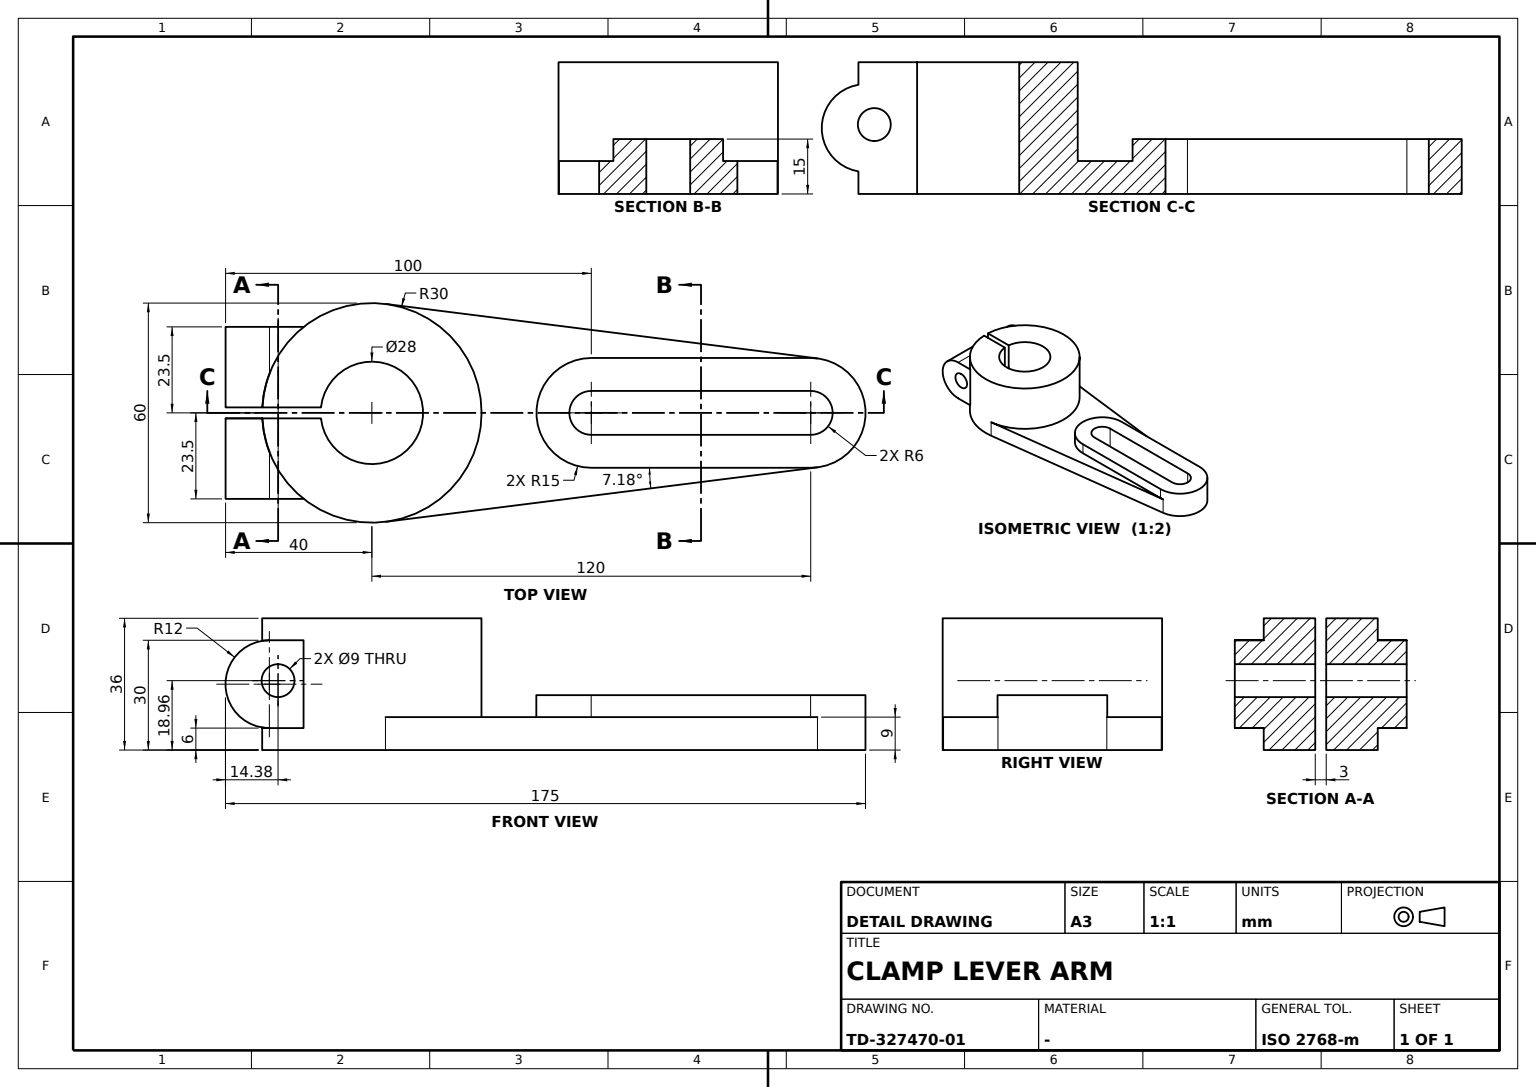
ISO-10303-21;
HEADER;
FILE_DESCRIPTION((''),'2;1');
FILE_NAME('','',(''),(''),'','','');
FILE_SCHEMA(('AUTOMOTIVE_DESIGN'));
ENDSEC;
DATA;
#1=APPLICATION_CONTEXT('');
#2=PRODUCT_CONTEXT('',#1,'mechanical');
#3=PRODUCT('','','',(#2));
#4=PRODUCT_DEFINITION_FORMATION('','',#3);
#5=PRODUCT_DEFINITION_CONTEXT('',#1,'design');
#6=PRODUCT_DEFINITION('','',#4,#5);
#7=PRODUCT_DEFINITION_SHAPE('','',#6);
#8=(LENGTH_UNIT()NAMED_UNIT(*)SI_UNIT(.MILLI.,.METRE.));
#9=(NAMED_UNIT(*)PLANE_ANGLE_UNIT()SI_UNIT($,.RADIAN.));
#10=(NAMED_UNIT(*)SI_UNIT($,.STERADIAN.)SOLID_ANGLE_UNIT());
#11=UNCERTAINTY_MEASURE_WITH_UNIT(LENGTH_MEASURE(0.005),#8,'distance_accuracy_value','');
#12=(GEOMETRIC_REPRESENTATION_CONTEXT(3)GLOBAL_UNCERTAINTY_ASSIGNED_CONTEXT((#11))GLOBAL_UNIT_ASSIGNED_CONTEXT((#8,#9,#10))REPRESENTATION_CONTEXT('',''));
#13=CARTESIAN_POINT('',(-28.,-23.5,30.));
#14=VERTEX_POINT('',#13);
#15=CARTESIAN_POINT('',(-18.648056,-23.5,30.));
#16=VERTEX_POINT('',#15);
#17=CARTESIAN_POINT('',(0.,-23.5,30.));
#18=DIRECTION('',(1.,0.,0.));
#19=VECTOR('',#18,1000.);
#20=LINE('',#17,#19);
#21=EDGE_CURVE('',#14,#16,#20,.T.);
#22=ORIENTED_EDGE('',*,*,#21,.T.);
#23=CARTESIAN_POINT('',(-28.,-10.77033,30.));
#24=VERTEX_POINT('',#23);
#25=CARTESIAN_POINT('',(0.,0.,30.));
#26=DIRECTION('',(0.,0.,1.));
#27=AXIS2_PLACEMENT_3D('',#25,#26,#18);
#28=CIRCLE('',#27,30.);
#29=EDGE_CURVE('',#24,#16,#28,.T.);
#30=ORIENTED_EDGE('',*,*,#29,.F.);
#31=CARTESIAN_POINT('',(-28.,11.75,30.));
#32=DIRECTION('',(0.,1.,0.));
#33=VECTOR('',#32,1000.);
#34=LINE('',#31,#33);
#35=EDGE_CURVE('',#24,#14,#34,.F.);
#36=ORIENTED_EDGE('',*,*,#35,.T.);
#37=EDGE_LOOP('',(#22,#30,#36));
#38=FACE_BOUND('',#37,.T.);
#39=CARTESIAN_POINT('',(-28.,0.,30.));
#40=AXIS2_PLACEMENT_3D('',#39,#26,#18);
#41=PLANE('',#40);
#42=ADVANCED_FACE('',(#38),#41,.T.);
#43=CARTESIAN_POINT('',(3.75,29.764702,9.));
#44=VERTEX_POINT('',#43);
#45=CARTESIAN_POINT('',(3.75,-29.764702,9.));
#46=VERTEX_POINT('',#45);
#47=CARTESIAN_POINT('',(0.,0.,9.));
#48=DIRECTION('',(0.,0.,-1.));
#49=DIRECTION('',(-1.,0.,0.));
#50=AXIS2_PLACEMENT_3D('',#47,#48,#49);
#51=CIRCLE('',#50,30.);
#52=EDGE_CURVE('',#44,#46,#51,.T.);
#53=ORIENTED_EDGE('',*,*,#52,.F.);
#54=CARTESIAN_POINT('',(3.75,29.764702,0.));
#55=VERTEX_POINT('',#54);
#56=CARTESIAN_POINT('',(3.75,29.764702,18.));
#57=VECTOR('',#26,1000.);
#58=LINE('',#56,#57);
#59=EDGE_CURVE('',#55,#44,#58,.T.);
#60=ORIENTED_EDGE('',*,*,#59,.F.);
#61=CARTESIAN_POINT('',(-29.962476,1.5,0.));
#62=VERTEX_POINT('',#61);
#63=CARTESIAN_POINT('',(0.,0.,0.));
#64=AXIS2_PLACEMENT_3D('',#63,#26,#18);
#65=CIRCLE('',#64,30.);
#66=EDGE_CURVE('',#55,#62,#65,.T.);
#67=ORIENTED_EDGE('',*,*,#66,.T.);
#68=CARTESIAN_POINT('',(-29.962476,1.5,6.161559));
#69=VERTEX_POINT('',#68);
#70=CARTESIAN_POINT('',(-29.962476,1.5,6.161558));
#71=LINE('',#70,#57);
#72=EDGE_CURVE('',#69,#62,#71,.F.);
#73=ORIENTED_EDGE('',*,*,#72,.F.);
#74=CARTESIAN_POINT('',(-28.,10.77033,6.));
#75=VERTEX_POINT('',#74);
#76=CARTESIAN_POINT('',(-29.962477,1.5,6.161559));
#77=CARTESIAN_POINT('',(-29.802516,4.695205,6.135042));
#78=CARTESIAN_POINT('',(-29.148715,7.783976,6.));
#79=B_SPLINE_CURVE_WITH_KNOTS('',3,(#76,#77,#78,#74),.UNSPECIFIED.,.F.,.F.,(4,4),(0.,0.009477153),.UNSPECIFIED.);
#80=EDGE_CURVE('',#75,#69,#79,.F.);
#81=ORIENTED_EDGE('',*,*,#80,.F.);
#82=CARTESIAN_POINT('',(-18.648056,23.5,6.));
#83=VERTEX_POINT('',#82);
#84=CARTESIAN_POINT('',(0.,0.,6.));
#85=AXIS2_PLACEMENT_3D('',#84,#26,#18);
#86=CIRCLE('',#85,30.);
#87=EDGE_CURVE('',#83,#75,#86,.T.);
#88=ORIENTED_EDGE('',*,*,#87,.F.);
#89=CARTESIAN_POINT('',(-18.648056,23.5,30.));
#90=VERTEX_POINT('',#89);
#91=LINE('',#82,#57);
#92=EDGE_CURVE('',#83,#90,#91,.T.);
#93=ORIENTED_EDGE('',*,*,#92,.T.);
#94=CARTESIAN_POINT('',(-28.,10.77033,30.));
#95=VERTEX_POINT('',#94);
#96=EDGE_CURVE('',#90,#95,#28,.T.);
#97=ORIENTED_EDGE('',*,*,#96,.T.);
#98=CARTESIAN_POINT('',(-29.962476,1.5,29.838441));
#99=VERTEX_POINT('',#98);
#100=CARTESIAN_POINT('',(-29.962477,1.5,29.838441));
#101=CARTESIAN_POINT('',(-29.802516,4.695205,29.864958));
#102=CARTESIAN_POINT('',(-29.148715,7.783976,30.));
#103=B_SPLINE_CURVE_WITH_KNOTS('',3,(#100,#101,#102,#94),.UNSPECIFIED.,.F.,.F.,(4,4),(0.,0.009477153),.UNSPECIFIED.);
#104=EDGE_CURVE('',#99,#95,#103,.T.);
#105=ORIENTED_EDGE('',*,*,#104,.F.);
#106=CARTESIAN_POINT('',(-29.962477,1.5,36.));
#107=VERTEX_POINT('',#106);
#108=LINE('',#106,#57);
#109=EDGE_CURVE('',#107,#99,#108,.F.);
#110=ORIENTED_EDGE('',*,*,#109,.F.);
#111=CARTESIAN_POINT('',(-29.962477,-1.5,36.));
#112=VERTEX_POINT('',#111);
#113=CARTESIAN_POINT('',(0.,0.,36.));
#114=AXIS2_PLACEMENT_3D('',#113,#26,#18);
#115=CIRCLE('',#114,30.);
#116=EDGE_CURVE('',#112,#107,#115,.T.);
#117=ORIENTED_EDGE('',*,*,#116,.F.);
#118=CARTESIAN_POINT('',(-29.962477,-1.5,29.838441));
#119=VERTEX_POINT('',#118);
#120=LINE('',#111,#57);
#121=EDGE_CURVE('',#112,#119,#120,.F.);
#122=ORIENTED_EDGE('',*,*,#121,.T.);
#123=CARTESIAN_POINT('',(-29.802516,-4.695205,29.864958));
#124=CARTESIAN_POINT('',(-29.148715,-7.783976,30.));
#125=B_SPLINE_CURVE_WITH_KNOTS('',3,(#118,#123,#124,#23),.UNSPECIFIED.,.F.,.F.,(4,4),(0.,0.009477153),.UNSPECIFIED.);
#126=EDGE_CURVE('',#24,#119,#125,.F.);
#127=ORIENTED_EDGE('',*,*,#126,.F.);
#128=ORIENTED_EDGE('',*,*,#29,.T.);
#129=CARTESIAN_POINT('',(-18.648056,-23.5,6.));
#130=VERTEX_POINT('',#129);
#131=LINE('',#129,#57);
#132=EDGE_CURVE('',#130,#16,#131,.T.);
#133=ORIENTED_EDGE('',*,*,#132,.F.);
#134=CARTESIAN_POINT('',(-28.,-10.77033,6.));
#135=VERTEX_POINT('',#134);
#136=EDGE_CURVE('',#135,#130,#86,.T.);
#137=ORIENTED_EDGE('',*,*,#136,.F.);
#138=CARTESIAN_POINT('',(-29.962476,-1.5,6.161559));
#139=VERTEX_POINT('',#138);
#140=CARTESIAN_POINT('',(-29.962477,-1.5,6.161559));
#141=CARTESIAN_POINT('',(-29.802516,-4.695205,6.135042));
#142=CARTESIAN_POINT('',(-29.148715,-7.783976,6.));
#143=B_SPLINE_CURVE_WITH_KNOTS('',3,(#140,#141,#142,#134),.UNSPECIFIED.,.F.,.F.,(4,4),(0.,0.009477153),.UNSPECIFIED.);
#144=EDGE_CURVE('',#139,#135,#143,.T.);
#145=ORIENTED_EDGE('',*,*,#144,.F.);
#146=CARTESIAN_POINT('',(-29.962476,-1.5,0.));
#147=VERTEX_POINT('',#146);
#148=CARTESIAN_POINT('',(-29.962476,-1.5,6.161558));
#149=LINE('',#148,#57);
#150=EDGE_CURVE('',#139,#147,#149,.F.);
#151=ORIENTED_EDGE('',*,*,#150,.T.);
#152=CARTESIAN_POINT('',(3.75,-29.764702,0.));
#153=VERTEX_POINT('',#152);
#154=EDGE_CURVE('',#147,#153,#65,.T.);
#155=ORIENTED_EDGE('',*,*,#154,.T.);
#156=CARTESIAN_POINT('',(3.75,-29.764702,18.));
#157=LINE('',#156,#57);
#158=EDGE_CURVE('',#153,#46,#157,.T.);
#159=ORIENTED_EDGE('',*,*,#158,.T.);
#160=EDGE_LOOP('',(#53,#60,#67,#73,#81,#88,#93,#97,#105,#110,#117,#122,#127,#128,#133,#137,#145,#151,#155,#159));
#161=FACE_BOUND('',#160,.T.);
#162=CARTESIAN_POINT('',(0.,0.,18.));
#163=AXIS2_PLACEMENT_3D('',#162,#26,#18);
#164=CYLINDRICAL_SURFACE('',#163,30.);
#165=ADVANCED_FACE('',(#161),#164,.T.);
#166=CARTESIAN_POINT('',(-28.,-23.5,6.));
#167=VERTEX_POINT('',#166);
#168=CARTESIAN_POINT('',(-28.,-23.5,18.));
#169=AXIS2_PLACEMENT_3D('',#168,#32,#26);
#170=CIRCLE('',#169,12.);
#171=EDGE_CURVE('',#167,#14,#170,.T.);
#172=ORIENTED_EDGE('',*,*,#171,.T.);
#173=ORIENTED_EDGE('',*,*,#35,.F.);
#174=ORIENTED_EDGE('',*,*,#126,.T.);
#175=CARTESIAN_POINT('',(-28.,-1.5,18.));
#176=AXIS2_PLACEMENT_3D('',#175,#32,#26);
#177=CIRCLE('',#176,12.);
#178=EDGE_CURVE('',#139,#119,#177,.T.);
#179=ORIENTED_EDGE('',*,*,#178,.F.);
#180=ORIENTED_EDGE('',*,*,#144,.T.);
#181=CARTESIAN_POINT('',(-28.,11.75,6.));
#182=LINE('',#181,#33);
#183=EDGE_CURVE('',#135,#167,#182,.F.);
#184=ORIENTED_EDGE('',*,*,#183,.T.);
#185=EDGE_LOOP('',(#172,#173,#174,#179,#180,#184));
#186=FACE_BOUND('',#185,.T.);
#187=CARTESIAN_POINT('',(-28.,11.75,18.));
#188=AXIS2_PLACEMENT_3D('',#187,#32,#49);
#189=CYLINDRICAL_SURFACE('',#188,12.);
#190=ADVANCED_FACE('',(#186),#189,.T.);
#191=CARTESIAN_POINT('',(120.,-15.,9.));
#192=VERTEX_POINT('',#191);
#193=CARTESIAN_POINT('',(120.,-15.,15.));
#194=VERTEX_POINT('',#193);
#195=CARTESIAN_POINT('',(120.,-15.,7.5));
#196=LINE('',#195,#57);
#197=EDGE_CURVE('',#192,#194,#196,.T.);
#198=ORIENTED_EDGE('',*,*,#197,.F.);
#199=CARTESIAN_POINT('',(121.875,-14.882351,9.));
#200=VERTEX_POINT('',#199);
#201=CARTESIAN_POINT('',(120.,0.,9.));
#202=AXIS2_PLACEMENT_3D('',#201,#48,#49);
#203=CIRCLE('',#202,15.);
#204=EDGE_CURVE('',#200,#192,#203,.T.);
#205=ORIENTED_EDGE('',*,*,#204,.F.);
#206=CARTESIAN_POINT('',(121.875,-14.882351,0.));
#207=VERTEX_POINT('',#206);
#208=CARTESIAN_POINT('',(121.875,-14.882351,7.5));
#209=LINE('',#208,#57);
#210=EDGE_CURVE('',#207,#200,#209,.T.);
#211=ORIENTED_EDGE('',*,*,#210,.F.);
#212=CARTESIAN_POINT('',(121.875,14.882351,0.));
#213=VERTEX_POINT('',#212);
#214=CARTESIAN_POINT('',(120.,0.,0.));
#215=AXIS2_PLACEMENT_3D('',#214,#26,#18);
#216=CIRCLE('',#215,15.);
#217=EDGE_CURVE('',#207,#213,#216,.T.);
#218=ORIENTED_EDGE('',*,*,#217,.T.);
#219=CARTESIAN_POINT('',(121.875,14.882351,9.));
#220=VERTEX_POINT('',#219);
#221=CARTESIAN_POINT('',(121.875,14.882351,7.5));
#222=LINE('',#221,#57);
#223=EDGE_CURVE('',#213,#220,#222,.T.);
#224=ORIENTED_EDGE('',*,*,#223,.T.);
#225=CARTESIAN_POINT('',(120.,15.,9.));
#226=VERTEX_POINT('',#225);
#227=EDGE_CURVE('',#226,#220,#203,.T.);
#228=ORIENTED_EDGE('',*,*,#227,.F.);
#229=CARTESIAN_POINT('',(120.,15.,15.));
#230=VERTEX_POINT('',#229);
#231=CARTESIAN_POINT('',(120.,15.,7.5));
#232=LINE('',#231,#57);
#233=EDGE_CURVE('',#226,#230,#232,.T.);
#234=ORIENTED_EDGE('',*,*,#233,.T.);
#235=CARTESIAN_POINT('',(120.,0.,15.));
#236=AXIS2_PLACEMENT_3D('',#235,#26,#18);
#237=CIRCLE('',#236,15.);
#238=EDGE_CURVE('',#194,#230,#237,.T.);
#239=ORIENTED_EDGE('',*,*,#238,.F.);
#240=EDGE_LOOP('',(#198,#205,#211,#218,#224,#228,#234,#239));
#241=FACE_BOUND('',#240,.T.);
#242=CARTESIAN_POINT('',(120.,0.,7.5));
#243=AXIS2_PLACEMENT_3D('',#242,#26,#18);
#244=CYLINDRICAL_SURFACE('',#243,15.);
#245=ADVANCED_FACE('',(#241),#244,.T.);
#246=ORIENTED_EDGE('',*,*,#227,.T.);
#247=DIRECTION('',(0.992156742,-0.125,0.));
#248=VECTOR('',#247,1000.);
#249=LINE('',#43,#248);
#250=EDGE_CURVE('',#44,#220,#249,.T.);
#251=ORIENTED_EDGE('',*,*,#250,.F.);
#252=ORIENTED_EDGE('',*,*,#52,.T.);
#253=DIRECTION('',(0.992156742,0.125,0.));
#254=VECTOR('',#253,1000.);
#255=LINE('',#45,#254);
#256=EDGE_CURVE('',#46,#200,#255,.T.);
#257=ORIENTED_EDGE('',*,*,#256,.T.);
#258=ORIENTED_EDGE('',*,*,#204,.T.);
#259=CARTESIAN_POINT('',(60.,-15.,9.));
#260=VERTEX_POINT('',#259);
#261=CARTESIAN_POINT('',(0.,-15.,9.));
#262=LINE('',#261,#19);
#263=EDGE_CURVE('',#260,#192,#262,.T.);
#264=ORIENTED_EDGE('',*,*,#263,.F.);
#265=CARTESIAN_POINT('',(60.,15.,9.));
#266=VERTEX_POINT('',#265);
#267=CARTESIAN_POINT('',(60.,0.,9.));
#268=AXIS2_PLACEMENT_3D('',#267,#48,#49);
#269=CIRCLE('',#268,15.);
#270=EDGE_CURVE('',#260,#266,#269,.T.);
#271=ORIENTED_EDGE('',*,*,#270,.T.);
#272=CARTESIAN_POINT('',(0.,15.,9.));
#273=VECTOR('',#49,1000.);
#274=LINE('',#272,#273);
#275=EDGE_CURVE('',#226,#266,#274,.T.);
#276=ORIENTED_EDGE('',*,*,#275,.F.);
#277=EDGE_LOOP('',(#246,#251,#252,#257,#258,#264,#271,#276));
#278=FACE_BOUND('',#277,.T.);
#279=AXIS2_PLACEMENT_3D('',#47,#48,#18);
#280=PLANE('',#279);
#281=ADVANCED_FACE('',(#278),#280,.F.);
#282=CARTESIAN_POINT('',(-13.919411,1.5,36.));
#283=VERTEX_POINT('',#282);
#284=CARTESIAN_POINT('',(-13.919411,1.5,0.));
#285=VERTEX_POINT('',#284);
#286=CARTESIAN_POINT('',(-13.919411,1.5,30.));
#287=LINE('',#286,#57);
#288=EDGE_CURVE('',#283,#285,#287,.F.);
#289=ORIENTED_EDGE('',*,*,#288,.T.);
#290=CARTESIAN_POINT('',(-13.919411,-1.5,0.));
#291=VERTEX_POINT('',#290);
#292=CIRCLE('',#64,14.);
#293=EDGE_CURVE('',#291,#285,#292,.T.);
#294=ORIENTED_EDGE('',*,*,#293,.F.);
#295=CARTESIAN_POINT('',(-13.919411,-1.5,36.));
#296=VERTEX_POINT('',#295);
#297=CARTESIAN_POINT('',(-13.919411,-1.5,30.));
#298=LINE('',#297,#57);
#299=EDGE_CURVE('',#291,#296,#298,.T.);
#300=ORIENTED_EDGE('',*,*,#299,.T.);
#301=CIRCLE('',#114,14.);
#302=EDGE_CURVE('',#296,#283,#301,.T.);
#303=ORIENTED_EDGE('',*,*,#302,.T.);
#304=EDGE_LOOP('',(#289,#294,#300,#303));
#305=FACE_BOUND('',#304,.T.);
#306=CARTESIAN_POINT('',(0.,0.,17.34));
#307=AXIS2_PLACEMENT_3D('',#306,#26,#18);
#308=CYLINDRICAL_SURFACE('',#307,14.);
#309=ADVANCED_FACE('',(#305),#308,.F.);
#310=CARTESIAN_POINT('',(120.,-6.,0.));
#311=VERTEX_POINT('',#310);
#312=CARTESIAN_POINT('',(120.,6.,0.));
#313=VERTEX_POINT('',#312);
#314=CIRCLE('',#215,6.);
#315=EDGE_CURVE('',#311,#313,#314,.T.);
#316=ORIENTED_EDGE('',*,*,#315,.T.);
#317=CARTESIAN_POINT('',(60.,6.,0.));
#318=VERTEX_POINT('',#317);
#319=CARTESIAN_POINT('',(0.,6.,0.));
#320=LINE('',#319,#19);
#321=EDGE_CURVE('',#318,#313,#320,.T.);
#322=ORIENTED_EDGE('',*,*,#321,.F.);
#323=CARTESIAN_POINT('',(60.,-6.,0.));
#324=VERTEX_POINT('',#323);
#325=CARTESIAN_POINT('',(60.,0.,0.));
#326=AXIS2_PLACEMENT_3D('',#325,#26,#18);
#327=CIRCLE('',#326,6.);
#328=EDGE_CURVE('',#318,#324,#327,.T.);
#329=ORIENTED_EDGE('',*,*,#328,.T.);
#330=CARTESIAN_POINT('',(0.,-6.,0.));
#331=LINE('',#330,#273);
#332=EDGE_CURVE('',#311,#324,#331,.T.);
#333=ORIENTED_EDGE('',*,*,#332,.F.);
#334=EDGE_LOOP('',(#316,#322,#329,#333));
#335=FACE_BOUND('',#334,.T.);
#336=LINE('',#152,#254);
#337=EDGE_CURVE('',#153,#207,#336,.T.);
#338=ORIENTED_EDGE('',*,*,#337,.F.);
#339=ORIENTED_EDGE('',*,*,#154,.F.);
#340=CARTESIAN_POINT('',(0.,-1.5,0.));
#341=LINE('',#340,#273);
#342=EDGE_CURVE('',#291,#147,#341,.T.);
#343=ORIENTED_EDGE('',*,*,#342,.F.);
#344=ORIENTED_EDGE('',*,*,#293,.T.);
#345=LINE('',#284,#273);
#346=EDGE_CURVE('',#285,#62,#345,.T.);
#347=ORIENTED_EDGE('',*,*,#346,.T.);
#348=ORIENTED_EDGE('',*,*,#66,.F.);
#349=LINE('',#54,#248);
#350=EDGE_CURVE('',#55,#213,#349,.T.);
#351=ORIENTED_EDGE('',*,*,#350,.T.);
#352=ORIENTED_EDGE('',*,*,#217,.F.);
#353=EDGE_LOOP('',(#338,#339,#343,#344,#347,#348,#351,#352));
#354=FACE_BOUND('',#353,.T.);
#355=PLANE('',#64);
#356=ADVANCED_FACE('',(#335,#354),#355,.F.);
#357=CARTESIAN_POINT('',(-25.620803,23.5,23.464319));
#358=VERTEX_POINT('',#357);
#359=CARTESIAN_POINT('',(-25.620803,23.5,18.964319));
#360=AXIS2_PLACEMENT_3D('',#359,#32,#26);
#361=CIRCLE('',#360,4.5);
#362=EDGE_CURVE('',#358,#358,#361,.T.);
#363=ORIENTED_EDGE('',*,*,#362,.T.);
#364=EDGE_LOOP('',(#363));
#365=FACE_BOUND('',#364,.T.);
#366=CARTESIAN_POINT('',(-25.620803,1.5,14.464319));
#367=VERTEX_POINT('',#366);
#368=CARTESIAN_POINT('',(-25.620803,1.5,18.964319));
#369=DIRECTION('',(0.,-1.,0.));
#370=AXIS2_PLACEMENT_3D('',#368,#369,#48);
#371=CIRCLE('',#370,4.5);
#372=EDGE_CURVE('',#367,#367,#371,.T.);
#373=ORIENTED_EDGE('',*,*,#372,.T.);
#374=EDGE_LOOP('',(#373));
#375=FACE_BOUND('',#374,.T.);
#376=CARTESIAN_POINT('',(-25.620803,3.91,18.964319));
#377=AXIS2_PLACEMENT_3D('',#376,#369,#18);
#378=CYLINDRICAL_SURFACE('',#377,4.5);
#379=ADVANCED_FACE('',(#365,#375),#378,.F.);
#380=CARTESIAN_POINT('',(60.,15.,15.));
#381=VERTEX_POINT('',#380);
#382=CARTESIAN_POINT('',(60.,-15.,15.));
#383=VERTEX_POINT('',#382);
#384=CARTESIAN_POINT('',(60.,0.,15.));
#385=AXIS2_PLACEMENT_3D('',#384,#26,#18);
#386=CIRCLE('',#385,15.);
#387=EDGE_CURVE('',#381,#383,#386,.T.);
#388=ORIENTED_EDGE('',*,*,#387,.F.);
#389=CARTESIAN_POINT('',(60.,15.,7.5));
#390=LINE('',#389,#57);
#391=EDGE_CURVE('',#266,#381,#390,.T.);
#392=ORIENTED_EDGE('',*,*,#391,.F.);
#393=ORIENTED_EDGE('',*,*,#270,.F.);
#394=CARTESIAN_POINT('',(60.,-15.,7.5));
#395=LINE('',#394,#57);
#396=EDGE_CURVE('',#260,#383,#395,.T.);
#397=ORIENTED_EDGE('',*,*,#396,.T.);
#398=EDGE_LOOP('',(#388,#392,#393,#397));
#399=FACE_BOUND('',#398,.T.);
#400=CARTESIAN_POINT('',(60.,0.,7.5));
#401=AXIS2_PLACEMENT_3D('',#400,#26,#18);
#402=CYLINDRICAL_SURFACE('',#401,15.);
#403=ADVANCED_FACE('',(#399),#402,.T.);
#404=CARTESIAN_POINT('',(60.,6.,15.));
#405=VERTEX_POINT('',#404);
#406=CARTESIAN_POINT('',(60.,6.,7.5));
#407=LINE('',#406,#57);
#408=EDGE_CURVE('',#318,#405,#407,.T.);
#409=ORIENTED_EDGE('',*,*,#408,.T.);
#410=CARTESIAN_POINT('',(60.,-6.,15.));
#411=VERTEX_POINT('',#410);
#412=CIRCLE('',#385,6.);
#413=EDGE_CURVE('',#405,#411,#412,.T.);
#414=ORIENTED_EDGE('',*,*,#413,.T.);
#415=CARTESIAN_POINT('',(60.,-6.,7.5));
#416=LINE('',#415,#57);
#417=EDGE_CURVE('',#324,#411,#416,.T.);
#418=ORIENTED_EDGE('',*,*,#417,.F.);
#419=ORIENTED_EDGE('',*,*,#328,.F.);
#420=EDGE_LOOP('',(#409,#414,#418,#419));
#421=FACE_BOUND('',#420,.T.);
#422=CYLINDRICAL_SURFACE('',#401,6.);
#423=ADVANCED_FACE('',(#421),#422,.F.);
#424=CARTESIAN_POINT('',(120.,-6.,15.));
#425=VERTEX_POINT('',#424);
#426=CARTESIAN_POINT('',(0.,-6.,15.));
#427=LINE('',#426,#273);
#428=EDGE_CURVE('',#425,#411,#427,.T.);
#429=ORIENTED_EDGE('',*,*,#428,.F.);
#430=CARTESIAN_POINT('',(120.,-6.,7.5));
#431=LINE('',#430,#57);
#432=EDGE_CURVE('',#311,#425,#431,.T.);
#433=ORIENTED_EDGE('',*,*,#432,.F.);
#434=ORIENTED_EDGE('',*,*,#332,.T.);
#435=ORIENTED_EDGE('',*,*,#417,.T.);
#436=EDGE_LOOP('',(#429,#433,#434,#435));
#437=FACE_BOUND('',#436,.T.);
#438=AXIS2_PLACEMENT_3D('',#310,#32,#49);
#439=PLANE('',#438);
#440=ADVANCED_FACE('',(#437),#439,.T.);
#441=ORIENTED_EDGE('',*,*,#362,.F.);
#442=EDGE_LOOP('',(#441));
#443=FACE_BOUND('',#442,.T.);
#444=ORIENTED_EDGE('',*,*,#92,.F.);
#445=CARTESIAN_POINT('',(-28.,23.5,6.));
#446=VERTEX_POINT('',#445);
#447=CARTESIAN_POINT('',(0.,23.5,6.));
#448=LINE('',#447,#19);
#449=EDGE_CURVE('',#446,#83,#448,.T.);
#450=ORIENTED_EDGE('',*,*,#449,.F.);
#451=CARTESIAN_POINT('',(-28.,23.5,30.));
#452=VERTEX_POINT('',#451);
#453=CARTESIAN_POINT('',(-28.,23.5,18.));
#454=AXIS2_PLACEMENT_3D('',#453,#32,#26);
#455=CIRCLE('',#454,12.);
#456=EDGE_CURVE('',#446,#452,#455,.T.);
#457=ORIENTED_EDGE('',*,*,#456,.T.);
#458=CARTESIAN_POINT('',(0.,23.5,30.));
#459=LINE('',#458,#19);
#460=EDGE_CURVE('',#452,#90,#459,.T.);
#461=ORIENTED_EDGE('',*,*,#460,.T.);
#462=EDGE_LOOP('',(#444,#450,#457,#461));
#463=FACE_BOUND('',#462,.T.);
#464=CARTESIAN_POINT('',(0.,23.5,0.));
#465=AXIS2_PLACEMENT_3D('',#464,#32,#49);
#466=PLANE('',#465);
#467=ADVANCED_FACE('',(#443,#463),#466,.T.);
#468=ORIENTED_EDGE('',*,*,#396,.F.);
#469=ORIENTED_EDGE('',*,*,#263,.T.);
#470=ORIENTED_EDGE('',*,*,#197,.T.);
#471=CARTESIAN_POINT('',(0.,-15.,15.));
#472=LINE('',#471,#273);
#473=EDGE_CURVE('',#194,#383,#472,.T.);
#474=ORIENTED_EDGE('',*,*,#473,.T.);
#475=EDGE_LOOP('',(#468,#469,#470,#474));
#476=FACE_BOUND('',#475,.T.);
#477=CARTESIAN_POINT('',(120.,-15.,0.));
#478=AXIS2_PLACEMENT_3D('',#477,#32,#49);
#479=PLANE('',#478);
#480=ADVANCED_FACE('',(#476),#479,.F.);
#481=CARTESIAN_POINT('',(0.,-23.5,6.));
#482=LINE('',#481,#19);
#483=EDGE_CURVE('',#167,#130,#482,.T.);
#484=ORIENTED_EDGE('',*,*,#483,.F.);
#485=ORIENTED_EDGE('',*,*,#183,.F.);
#486=ORIENTED_EDGE('',*,*,#136,.T.);
#487=EDGE_LOOP('',(#484,#485,#486));
#488=FACE_BOUND('',#487,.T.);
#489=CARTESIAN_POINT('',(-28.,0.,6.));
#490=AXIS2_PLACEMENT_3D('',#489,#26,#18);
#491=PLANE('',#490);
#492=ADVANCED_FACE('',(#488),#491,.F.);
#493=ORIENTED_EDGE('',*,*,#408,.F.);
#494=ORIENTED_EDGE('',*,*,#321,.T.);
#495=CARTESIAN_POINT('',(120.,6.,15.));
#496=VERTEX_POINT('',#495);
#497=CARTESIAN_POINT('',(120.,6.,7.5));
#498=LINE('',#497,#57);
#499=EDGE_CURVE('',#313,#496,#498,.T.);
#500=ORIENTED_EDGE('',*,*,#499,.T.);
#501=CARTESIAN_POINT('',(0.,6.,15.));
#502=LINE('',#501,#19);
#503=EDGE_CURVE('',#405,#496,#502,.T.);
#504=ORIENTED_EDGE('',*,*,#503,.F.);
#505=EDGE_LOOP('',(#493,#494,#500,#504));
#506=FACE_BOUND('',#505,.T.);
#507=AXIS2_PLACEMENT_3D('',#317,#369,#18);
#508=PLANE('',#507);
#509=ADVANCED_FACE('',(#506),#508,.T.);
#510=CARTESIAN_POINT('',(-25.620803,-1.5,23.464319));
#511=VERTEX_POINT('',#510);
#512=CARTESIAN_POINT('',(-25.620803,-1.5,18.964319));
#513=AXIS2_PLACEMENT_3D('',#512,#32,#26);
#514=CIRCLE('',#513,4.5);
#515=EDGE_CURVE('',#511,#511,#514,.T.);
#516=ORIENTED_EDGE('',*,*,#515,.T.);
#517=EDGE_LOOP('',(#516));
#518=FACE_BOUND('',#517,.T.);
#519=CARTESIAN_POINT('',(-25.620803,-23.5,23.464319));
#520=VERTEX_POINT('',#519);
#521=CARTESIAN_POINT('',(-25.620803,-23.5,18.964319));
#522=AXIS2_PLACEMENT_3D('',#521,#32,#26);
#523=CIRCLE('',#522,4.5);
#524=EDGE_CURVE('',#520,#520,#523,.F.);
#525=ORIENTED_EDGE('',*,*,#524,.T.);
#526=EDGE_LOOP('',(#525));
#527=FACE_BOUND('',#526,.T.);
#528=ADVANCED_FACE('',(#518,#527),#378,.F.);
#529=ORIENTED_EDGE('',*,*,#233,.F.);
#530=ORIENTED_EDGE('',*,*,#275,.T.);
#531=ORIENTED_EDGE('',*,*,#391,.T.);
#532=CARTESIAN_POINT('',(0.,15.,15.));
#533=LINE('',#532,#19);
#534=EDGE_CURVE('',#381,#230,#533,.T.);
#535=ORIENTED_EDGE('',*,*,#534,.T.);
#536=EDGE_LOOP('',(#529,#530,#531,#535));
#537=FACE_BOUND('',#536,.T.);
#538=CARTESIAN_POINT('',(60.,15.,0.));
#539=AXIS2_PLACEMENT_3D('',#538,#369,#18);
#540=PLANE('',#539);
#541=ADVANCED_FACE('',(#537),#540,.F.);
#542=ORIENTED_EDGE('',*,*,#515,.F.);
#543=EDGE_LOOP('',(#542));
#544=FACE_BOUND('',#543,.T.);
#545=ORIENTED_EDGE('',*,*,#299,.F.);
#546=ORIENTED_EDGE('',*,*,#342,.T.);
#547=ORIENTED_EDGE('',*,*,#150,.F.);
#548=ORIENTED_EDGE('',*,*,#178,.T.);
#549=ORIENTED_EDGE('',*,*,#121,.F.);
#550=CARTESIAN_POINT('',(-50.,-1.5,36.));
#551=LINE('',#550,#19);
#552=EDGE_CURVE('',#112,#296,#551,.T.);
#553=ORIENTED_EDGE('',*,*,#552,.T.);
#554=EDGE_LOOP('',(#545,#546,#547,#548,#549,#553));
#555=FACE_BOUND('',#554,.T.);
#556=AXIS2_PLACEMENT_3D('',#550,#32,#18);
#557=PLANE('',#556);
#558=ADVANCED_FACE('',(#544,#555),#557,.T.);
#559=ORIENTED_EDGE('',*,*,#483,.T.);
#560=ORIENTED_EDGE('',*,*,#132,.T.);
#561=ORIENTED_EDGE('',*,*,#21,.F.);
#562=ORIENTED_EDGE('',*,*,#171,.F.);
#563=EDGE_LOOP('',(#559,#560,#561,#562));
#564=FACE_BOUND('',#563,.T.);
#565=ORIENTED_EDGE('',*,*,#524,.F.);
#566=EDGE_LOOP('',(#565));
#567=FACE_BOUND('',#566,.T.);
#568=CARTESIAN_POINT('',(0.,-23.5,0.));
#569=AXIS2_PLACEMENT_3D('',#568,#32,#49);
#570=PLANE('',#569);
#571=ADVANCED_FACE('',(#564,#567),#570,.F.);
#572=ORIENTED_EDGE('',*,*,#96,.F.);
#573=ORIENTED_EDGE('',*,*,#460,.F.);
#574=EDGE_CURVE('',#95,#452,#34,.T.);
#575=ORIENTED_EDGE('',*,*,#574,.F.);
#576=EDGE_LOOP('',(#572,#573,#575));
#577=FACE_BOUND('',#576,.T.);
#578=ADVANCED_FACE('',(#577),#41,.T.);
#579=ORIENTED_EDGE('',*,*,#387,.T.);
#580=ORIENTED_EDGE('',*,*,#473,.F.);
#581=ORIENTED_EDGE('',*,*,#238,.T.);
#582=ORIENTED_EDGE('',*,*,#534,.F.);
#583=EDGE_LOOP('',(#579,#580,#581,#582));
#584=FACE_BOUND('',#583,.T.);
#585=CIRCLE('',#236,6.);
#586=EDGE_CURVE('',#425,#496,#585,.T.);
#587=ORIENTED_EDGE('',*,*,#586,.F.);
#588=ORIENTED_EDGE('',*,*,#428,.T.);
#589=ORIENTED_EDGE('',*,*,#413,.F.);
#590=ORIENTED_EDGE('',*,*,#503,.T.);
#591=EDGE_LOOP('',(#587,#588,#589,#590));
#592=FACE_BOUND('',#591,.T.);
#593=CARTESIAN_POINT('',(0.,0.,15.));
#594=AXIS2_PLACEMENT_3D('',#593,#26,#18);
#595=PLANE('',#594);
#596=ADVANCED_FACE('',(#584,#592),#595,.T.);
#597=ORIENTED_EDGE('',*,*,#586,.T.);
#598=ORIENTED_EDGE('',*,*,#499,.F.);
#599=ORIENTED_EDGE('',*,*,#315,.F.);
#600=ORIENTED_EDGE('',*,*,#432,.T.);
#601=EDGE_LOOP('',(#597,#598,#599,#600));
#602=FACE_BOUND('',#601,.T.);
#603=CYLINDRICAL_SURFACE('',#243,6.);
#604=ADVANCED_FACE('',(#602),#603,.F.);
#605=ORIENTED_EDGE('',*,*,#210,.T.);
#606=ORIENTED_EDGE('',*,*,#256,.F.);
#607=ORIENTED_EDGE('',*,*,#158,.F.);
#608=ORIENTED_EDGE('',*,*,#337,.T.);
#609=EDGE_LOOP('',(#605,#606,#607,#608));
#610=FACE_BOUND('',#609,.T.);
#611=DIRECTION('',(0.125,-0.992156742,0.));
#612=AXIS2_PLACEMENT_3D('',#152,#611,#253);
#613=PLANE('',#612);
#614=ADVANCED_FACE('',(#610),#613,.T.);
#615=ORIENTED_EDGE('',*,*,#302,.F.);
#616=ORIENTED_EDGE('',*,*,#552,.F.);
#617=ORIENTED_EDGE('',*,*,#116,.T.);
#618=LINE('',#282,#273);
#619=EDGE_CURVE('',#283,#107,#618,.T.);
#620=ORIENTED_EDGE('',*,*,#619,.F.);
#621=EDGE_LOOP('',(#615,#616,#617,#620));
#622=FACE_BOUND('',#621,.T.);
#623=PLANE('',#114);
#624=ADVANCED_FACE('',(#622),#623,.T.);
#625=CARTESIAN_POINT('',(-28.,1.5,18.));
#626=AXIS2_PLACEMENT_3D('',#625,#369,#48);
#627=CIRCLE('',#626,12.);
#628=EDGE_CURVE('',#99,#69,#627,.T.);
#629=ORIENTED_EDGE('',*,*,#628,.F.);
#630=ORIENTED_EDGE('',*,*,#104,.T.);
#631=ORIENTED_EDGE('',*,*,#574,.T.);
#632=ORIENTED_EDGE('',*,*,#456,.F.);
#633=EDGE_CURVE('',#75,#446,#182,.T.);
#634=ORIENTED_EDGE('',*,*,#633,.F.);
#635=ORIENTED_EDGE('',*,*,#80,.T.);
#636=EDGE_LOOP('',(#629,#630,#631,#632,#634,#635));
#637=FACE_BOUND('',#636,.T.);
#638=ADVANCED_FACE('',(#637),#189,.T.);
#639=ORIENTED_EDGE('',*,*,#449,.T.);
#640=ORIENTED_EDGE('',*,*,#87,.T.);
#641=ORIENTED_EDGE('',*,*,#633,.T.);
#642=EDGE_LOOP('',(#639,#640,#641));
#643=FACE_BOUND('',#642,.T.);
#644=ADVANCED_FACE('',(#643),#491,.F.);
#645=ORIENTED_EDGE('',*,*,#59,.T.);
#646=ORIENTED_EDGE('',*,*,#250,.T.);
#647=ORIENTED_EDGE('',*,*,#223,.F.);
#648=ORIENTED_EDGE('',*,*,#350,.F.);
#649=EDGE_LOOP('',(#645,#646,#647,#648));
#650=FACE_BOUND('',#649,.T.);
#651=DIRECTION('',(-0.125,-0.992156742,0.));
#652=AXIS2_PLACEMENT_3D('',#54,#651,#247);
#653=PLANE('',#652);
#654=ADVANCED_FACE('',(#650),#653,.F.);
#655=ORIENTED_EDGE('',*,*,#628,.T.);
#656=ORIENTED_EDGE('',*,*,#72,.T.);
#657=ORIENTED_EDGE('',*,*,#346,.F.);
#658=ORIENTED_EDGE('',*,*,#288,.F.);
#659=ORIENTED_EDGE('',*,*,#619,.T.);
#660=ORIENTED_EDGE('',*,*,#109,.T.);
#661=EDGE_LOOP('',(#655,#656,#657,#658,#659,#660));
#662=FACE_BOUND('',#661,.T.);
#663=ORIENTED_EDGE('',*,*,#372,.F.);
#664=EDGE_LOOP('',(#663));
#665=FACE_BOUND('',#664,.T.);
#666=AXIS2_PLACEMENT_3D('',#282,#369,#49);
#667=PLANE('',#666);
#668=ADVANCED_FACE('',(#662,#665),#667,.T.);
#669=CLOSED_SHELL('',(#42,#165,#190,#245,#281,#309,#356,#379,#403,#423,#440,#467,#480,#492,#509,#528,#541,#558,#571,#578,#596,#604,#614,#624,#638,#644,#654,#668));
#670=MANIFOLD_SOLID_BREP('',#669);
#671=ADVANCED_BREP_SHAPE_REPRESENTATION('',(#670),#12);
#672=SHAPE_DEFINITION_REPRESENTATION(#7,#671);
ENDSEC;
END-ISO-10303-21;
